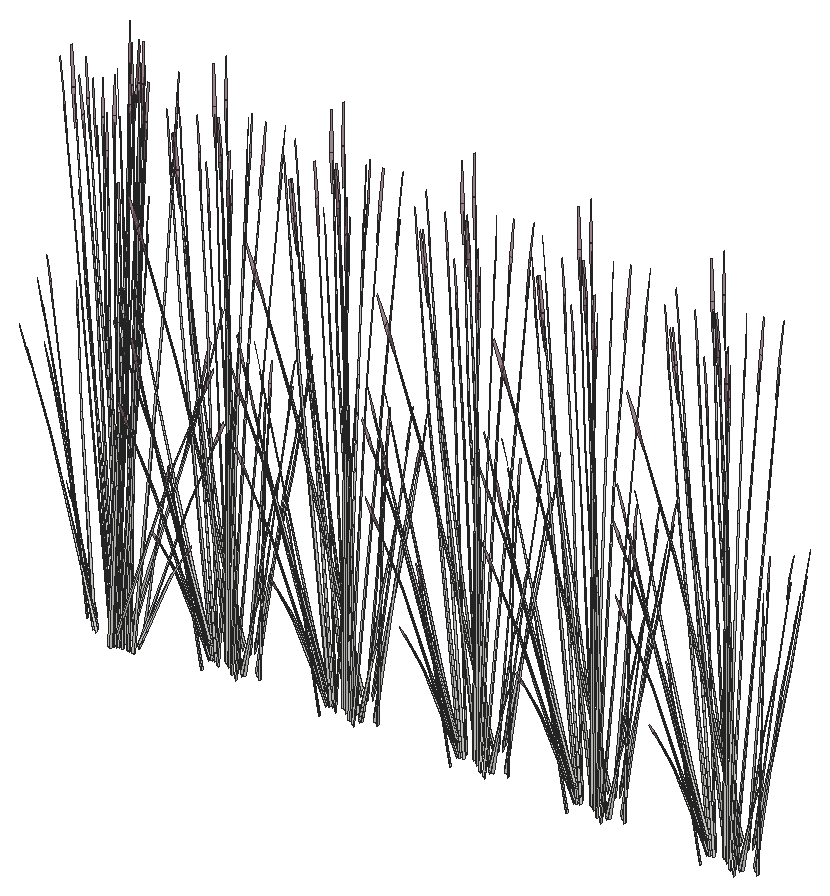
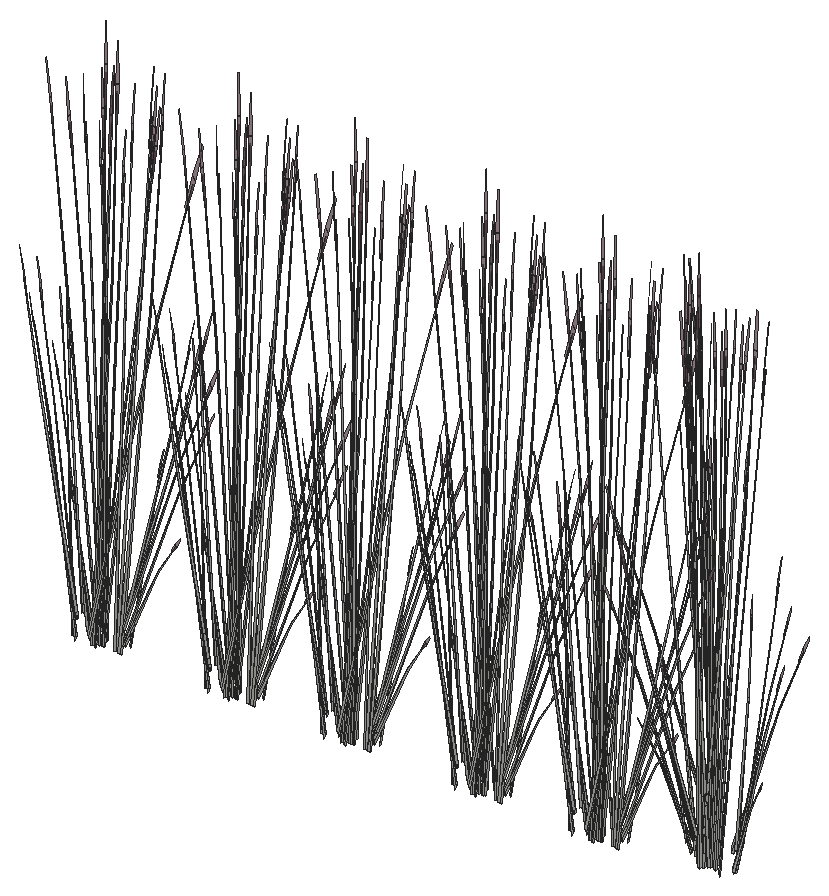
# SketchUp Ruby script. Lengths in inches.
U = 1.inch
M = Sketchup.active_model
def pt(a) = Geom::Point3d.new(a.map { |v| v * U })
def face(e, loops, mat)
  f = e.add_face(loops[0].map { |a| pt(a) })
  loops[1..].each { |l| e.add_face(l.map { |a| pt(a) }).erase! }
  f.material = f.back_material = mat if mat
  f
end
# faces: each face lists its corners as indices into pts; further lists are holes
def faces(e, pts, list, mat = nil) = list.each { |f| face(e, (f[0].is_a?(Array) ? f : [f]).map { |l| l.map { |i| pts[i] } }, mat) }
# xy, xz, yz: faces in a plane at the given z, y or x. An outline is a flat list of corners, or four numbers for a rectangle; further outlines are holes
def ring(l) = l.size == 4 ? [[l[0], l[1]], [l[2], l[1]], [l[2], l[3]], [l[0], l[3]]] : l.each_slice(2).to_a
def flat(e, list, mat, &to3) = list.each { |f| face(e, (f[0].is_a?(Array) ? f : [f]).map { |l| ring(l).map { |u, v| to3.(u, v) } }, mat) }
def xy(e, z, list, mat = nil) = flat(e, list, mat) { |x, y| [x, y, z] }
def xz(e, y, list, mat = nil) = flat(e, list, mat) { |x, z| [x, y, z] }
def yz(e, x, list, mat = nil) = flat(e, list, mat) { |y, z| [x, y, z] }
def lines(e, pts, list) = list.each { |a, b| e.add_line(pt(pts[a]), pt(pts[b])) }
# prism: a flat outline (further loops are holes) pulled along v
def prism(e, loops, v, mat = nil)
  f = face(e, loops, mat); d = Geom::Vector3d.new(v.map { |x| x * U })
  f.pushpull(f.normal.samedirection?(d) ? d.length : -d.length)
end
def box(e, o, s, mat = nil) = prism(e, [[o, [o[0] + s[0], o[1], o[2]], [o[0] + s[0], o[1] + s[1], o[2]], [o[0], o[1] + s[1], o[2]]]], [0, 0, s[2]], mat)
def at(x, y, z, deg = 0) = Geom::Transformation.translation(pt([x, y, z])) * Geom::Transformation.rotation(ORIGIN, Z_AXIS, deg.degrees)
def axes(o, x, y, z) = Geom::Transformation.new([*x, 0, *y, 0, *z, 0, *pt(o).to_a, 1])
def part(name) = M.definitions.add(name)
# library, detail: a bought-in or finely detailed component or shape, given as its bounding box
def library(name, o, s) = part(name).tap { |d| box(d.entities, o, s) }
def detail(e, o, s) = box(e.add_group.entities, o, s)
def put(e, d, t, mat = nil) = e.add_instance(d, t).tap { |i| i.material = mat if mat }
def group(e, t, mat = nil) = e.add_group.tap { |g| g.transformation = t; g.material = mat if mat }.entities
root = M.entities
M.materials.add("LightPink_Translucent").color = [144, 107, 117]
M.materials["LightPink_Translucent"].alpha = 0.75
c1 = part("blade")
p = [[2.15,0.21,22],[0,0.17,0],[0.09,0.45,0],[2.18,0.31,22],[2.29,0.31,22],[0.38,0.45,0],
  [2.48,0.24,33],[2.49,0.24,33],[2.48,0.22,33]]
faces(c1.entities,p,[[0,1,2,3],[4,5,2,3],[6,3,4,7],[8,0,3,6]])
c2 = part("seeds")
p = [[0.3,-0.1,1.38],[-0.01,-0.03,1.59],[-0.01,-0.03,0.03],[0.14,-0.07,-0.07],[0.29,-0.03,3],[0.15,0.01,3.11]]
faces(c2.entities,p,[[0,1,2,3],[1,0,4,5]],"LightPink_Translucent")
c3 = part("blade with seeds")
put(c3.entities,c1,at(0,0,0))
put(c3.entities,c2,axes([2.4,0.25,30.99],[1.5799,-0.05474,1.17369],[-0.12525,1.92788,0.29478],[-0.07173,-0.02425,1.56792]))
put(root,c3,axes([230.35,456.43,399.875],[-0.20841,0.0122,1.71376],[0.13825,-0.52864,0.13857],[0.297,0.0327,0.73262]))
put(root,c3,axes([229.68,456.33,398.38],[-0.63506,-0.11347,0.49198],[0.12924,-0.64083,0.19306],[0.09281,0.06188,1.70813]))
put(root,c3,axes([229.17,457.91,398.2],[-0.16394,-0.4643,0],[0.46814,-0.1626,0],[0,0,1.54371]))
put(root,c3,axes([228.86,457.47,398.62],[-0.09693,0.48062,0.1448],[-0.47357,-0.08343,-0.41347],[-0.08619,-0.04935,1.26744]))
put(root,c3,axes([240.53,461.875,399.33],[0.4342,0.21716,1.51261],[-0.42537,0.46784,0.59816],[-0.19053,-0.27728,1.26806]))
put(root,c3,axes([254.24,461.875,399.33],[0.4342,0.21716,1.51261],[-0.42537,0.46784,0.59816],[-0.19053,-0.27728,1.26806]))
put(root,c3,axes([269.49,461.875,399.33],[0.4342,0.21716,1.51261],[-0.42537,0.46784,0.59816],[-0.19053,-0.27728,1.26806]))
put(root,c3,axes([283.1,461.875,399.33],[0.4342,0.21716,1.51261],[-0.42537,0.46784,0.59816],[-0.19053,-0.27728,1.26806]))
put(root,c3,axes([298.63,461.875,399.33],[0.4342,0.21716,1.51261],[-0.42537,0.46784,0.59816],[-0.19053,-0.27728,1.26806]))
put(root,c3,axes([229.78,457.85,398.18],[0.5275,-0.18273,-0.19198],[0.18536,0.52636,0.00008],[0.05823,-0.0202,1.73897]))
put(root,c3,axes([229.97,458.07,398.47],[0.14515,-0.53522,0.17642],[0.53115,0.15146,0.35086],[-0.09175,0.00261,1.60407]))
put(root,c3,axes([242.61,459.71,398.59],[-0.1795,-0.01595,1.43002],[-0.18389,-0.42791,-0.30754],[0.22051,-0.12105,0.61141]))
put(root,c3,axes([256.32,459.71,398.59],[-0.1795,-0.01595,1.43002],[-0.18389,-0.42791,-0.30754],[0.22051,-0.12105,0.61141]))
put(root,c3,axes([271.57,459.71,398.59],[-0.1795,-0.01595,1.43002],[-0.18389,-0.42791,-0.30754],[0.22051,-0.12105,0.61141]))
put(root,c3,axes([285.18,459.71,398.59],[-0.1795,-0.01595,1.43002],[-0.18389,-0.42791,-0.30754],[0.22051,-0.12105,0.61141]))
put(root,c3,axes([300.71,459.71,398.59],[-0.1795,-0.01595,1.43002],[-0.18389,-0.42791,-0.30754],[0.22051,-0.12105,0.61141]))
put(root,c3,axes([229.84,456.85,398.21],[0.35073,0.34786,0],[-0.35073,0.34786,0],[0,0,1.69266]))
put(root,c3,axes([227.85,456.2,399.34],[0.14282,-0.0779,1.77064],[0.04925,0.54394,0.13857],[-0.30935,0.07218,0.63284]))
put(root,c3,axes([230.79,456.7,398.47],[-0.39477,-0.39228,0.17642],[0.39783,-0.38049,0.35086],[-0.0436,0.08011,1.60407]))
put(root,c3,axes([232.375,457.06,398.77],[-0.31044,0.08891,1.1486],[0.14613,-0.36744,0.84392],[0.16469,0.02514,0.25299]))
put(root,c3,axes([242.82,458.92,398.77],[-0.16736,0.27414,1.1486],[-0.14385,-0.36832,0.84392],[0.13822,-0.09229,0.25299]))
put(root,c3,axes([256.53,458.92,398.77],[-0.16736,0.27414,1.1486],[-0.14385,-0.36832,0.84392],[0.13822,-0.09229,0.25299]))
put(root,c3,axes([271.77,458.92,398.77],[-0.16736,0.27414,1.1486],[-0.14385,-0.36832,0.84392],[0.13822,-0.09229,0.25299]))
put(root,c3,axes([285.39,458.92,398.77],[-0.16736,0.27414,1.1486],[-0.14385,-0.36832,0.84392],[0.13822,-0.09229,0.25299]))
put(root,c3,axes([300.92,458.92,398.77],[-0.16736,0.27414,1.1486],[-0.14385,-0.36832,0.84392],[0.13822,-0.09229,0.25299]))
put(root,c3,axes([229.05,458.12,398.2],[-0.50654,-0.24178,0],[0.24378,-0.50239,0],[0,0,1.62707]))
put(root,c3,axes([229.47,457.48,398.46],[-0.49063,-0.43346,-0.25192],[0.41285,-0.48673,0.5513],[-0.13212,0.05071,1.68216]))
put(root,c3,axes([228.18,458.31,398.48],[0.47024,0.26927,0.49651],[-0.28107,0.48284,0],[-0.1071,-0.06133,1.57504]))
put(root,c3,axes([242.58,459.95,400.53],[0.43736,-0.07697,-0.35414],[0.11549,0.43998,0.4572],[0.12533,-0.11818,0.87481]))
put(root,c3,axes([256.29,459.95,400.53],[0.43736,-0.07697,-0.35414],[0.11549,0.43998,0.4572],[0.12533,-0.11818,0.87481]))
put(root,c3,axes([271.54,459.95,400.53],[0.43736,-0.07697,-0.35414],[0.11549,0.43998,0.4572],[0.12533,-0.11818,0.87481]))
put(root,c3,axes([285.15,459.95,400.53],[0.43736,-0.07697,-0.35414],[0.11549,0.43998,0.4572],[0.12533,-0.11818,0.87481]))
put(root,c3,axes([300.68,459.95,400.53],[0.43736,-0.07697,-0.35414],[0.11549,0.43998,0.4572],[0.12533,-0.11818,0.87481]))
put(root,c3,axes([229.84,456.45,398.72],[0.24378,-0.48527,0.44739],[0.50654,0.23354,-0.21531],[0,0.11186,1.43643]))
put(root,c3,axes([238.33,459.35,400.53],[-0.28589,-0.33718,-0.35414],[0.32644,-0.31919,0.4572],[-0.16586,-0.04856,0.87481]))
put(root,c3,axes([252.04,459.35,400.53],[-0.28589,-0.33718,-0.35414],[0.32644,-0.31919,0.4572],[-0.16586,-0.04856,0.87481]))
put(root,c3,axes([267.28,459.35,400.53],[-0.28589,-0.33718,-0.35414],[0.32644,-0.31919,0.4572],[-0.16586,-0.04856,0.87481]))
put(root,c3,axes([280.9,459.35,400.53],[-0.28589,-0.33718,-0.35414],[0.32644,-0.31919,0.4572],[-0.16586,-0.04856,0.87481]))
put(root,c3,axes([296.43,459.35,400.53],[-0.28589,-0.33718,-0.35414],[0.32644,-0.31919,0.4572],[-0.16586,-0.04856,0.87481]))
put(root,c3,axes([229.75,456.72,398.29],[0,0.62282,-0.05637],[-0.62828,0,0],[0,0.01957,1.79368]))
put(root,c3,axes([240.01,460.35,398.67],[-0.05855,-0.61451,-0.29095],[0.60981,-0.03716,-0.50002],[0.10738,-0.08185,1.59708]))
put(root,c3,axes([253.72,460.35,398.67],[-0.05855,-0.61451,-0.29095],[0.60981,-0.03716,-0.50002],[0.10738,-0.08185,1.59708]))
put(root,c3,axes([268.97,460.35,398.67],[-0.05855,-0.61451,-0.29095],[0.60981,-0.03716,-0.50002],[0.10738,-0.08185,1.59708]))
put(root,c3,axes([282.58,460.35,398.67],[-0.05855,-0.61451,-0.29095],[0.60981,-0.03716,-0.50002],[0.10738,-0.08185,1.59708]))
put(root,c3,axes([298.11,460.35,398.67],[-0.05855,-0.61451,-0.29095],[0.60981,-0.03716,-0.50002],[0.10738,-0.08185,1.59708]))
put(root,c3,axes([226.87,456.5,400.68],[-0.13612,0.48987,-0.51099],[-0.46669,-0.16791,-0.3958],[-0.1879,0.04492,0.97773]))
put(root,c3,axes([231.83,458.19,399.93],[-0.09617,-0.45271,-0.03492],[0.45453,-0.10408,-0.15832],[0.09492,0.0287,0.52218]))
put(root,c3,axes([227.91,458.59,398.375],[-0.31414,0.53965,0],[-0.52557,-0.30095,-0.51607],[-0.1197,-0.06854,1.63711]))
put(root,c3,axes([238.36,458.77,398.13],[-0.14494,0.43975,-0.03893],[-0.4461,-0.13527,-0.17649],[-0.06773,-0.07192,0.58215]))
put(root,c3,axes([252.07,458.77,398.13],[-0.14494,0.43975,-0.03893],[-0.4461,-0.13527,-0.17649],[-0.06773,-0.07192,0.58215]))
put(root,c3,axes([267.3125,458.77,398.13],[-0.14494,0.43975,-0.03893],[-0.4461,-0.13527,-0.17649],[-0.06773,-0.07192,0.58215]))
put(root,c3,axes([280.93,458.77,398.13],[-0.14494,0.43975,-0.03893],[-0.4461,-0.13527,-0.17649],[-0.06773,-0.07192,0.58215]))
put(root,c3,axes([296.46,458.77,398.13],[-0.14494,0.43975,-0.03893],[-0.4461,-0.13527,-0.17649],[-0.06773,-0.07192,0.58215]))
put(root,c3,axes([239.73,461,398.67],[-0.56585,-0.25696,-0.29095],[0.27246,-0.54236,-0.50002],[-0.01778,-0.13316,1.59708]))
put(root,c3,axes([253.4375,461,398.67],[-0.56585,-0.25696,-0.29095],[0.27246,-0.54236,-0.50002],[-0.01778,-0.13316,1.59708]))
put(root,c3,axes([268.68,461,398.67],[-0.56585,-0.25696,-0.29095],[0.27246,-0.54236,-0.50002],[-0.01778,-0.13316,1.59708]))
put(root,c3,axes([282.3,461,398.67],[-0.56585,-0.25696,-0.29095],[0.27246,-0.54236,-0.50002],[-0.01778,-0.13316,1.59708]))
put(root,c3,axes([297.83,461,398.67],[-0.56585,-0.25696,-0.29095],[0.27246,-0.54236,-0.50002],[-0.01778,-0.13316,1.59708]))
put(root,c3,axes([231.12,456.72,398.48],[0,-0.53854,0.49651],[0.56215,0,0],[0,0.12266,1.57504]))
put(root,c3,axes([238.12,460.78,398.375],[-0.62828,0,0],[0,-0.6019,-0.51607],[0,-0.13709,1.63711]))
put(root,c3,axes([251.83,460.78,398.375],[-0.62828,0,0],[0,-0.6019,-0.51607],[0,-0.13709,1.63711]))
put(root,c3,axes([267.07,460.78,398.375],[-0.62828,0,0],[0,-0.6019,-0.51607],[0,-0.13709,1.63711]))
put(root,c3,axes([280.6875,460.78,398.375],[-0.62828,0,0],[0,-0.6019,-0.51607],[0,-0.13709,1.63711]))
put(root,c3,axes([296.22,460.78,398.375],[-0.62828,0,0],[0,-0.6019,-0.51607],[0,-0.13709,1.63711]))
put(root,c3,axes([229.71,457.12,398.72],[0.54562,-0.03324,0.44739],[0.04934,0.55185,-0.21531],[-0.09768,0.05593,1.43643]))
put(root,c3,axes([230.05,456.56,398.62],[0.46814,-0.15705,0.1448],[0.16394,0.44848,-0.41347],[0,0.0987,1.26744]))
put(root,c3,axes([238.23,459.71,398.59],[0.0981,0.14994,1.43002],[-0.22605,0.40756,-0.30754],[-0.23211,-0.09741,0.61141]))
put(root,c3,axes([251.93,459.71,398.59],[0.0981,0.14994,1.43002],[-0.22605,0.40756,-0.30754],[-0.23211,-0.09741,0.61141]))
put(root,c3,axes([267.18,459.71,398.59],[0.0981,0.14994,1.43002],[-0.22605,0.40756,-0.30754],[-0.23211,-0.09741,0.61141]))
put(root,c3,axes([280.79,459.71,398.59],[0.0981,0.14994,1.43002],[-0.22605,0.40756,-0.30754],[-0.23211,-0.09741,0.61141]))
put(root,c3,axes([296.33,459.71,398.59],[0.0981,0.14994,1.43002],[-0.22605,0.40756,-0.30754],[-0.23211,-0.09741,0.61141]))
put(root,c3,axes([238.63,459.57,400.98],[-0.50227,-0.01297,-0.71045],[0.03373,-0.54602,0.08574],[-0.21278,-0.05762,1.00501]))
put(root,c3,axes([252.34,459.57,400.98],[-0.50227,-0.01297,-0.71045],[0.03373,-0.54602,0.08574],[-0.21278,-0.05762,1.00501]))
put(root,c3,axes([267.59,459.57,400.98],[-0.50227,-0.01297,-0.71045],[0.03373,-0.54602,0.08574],[-0.21278,-0.05762,1.00501]))
put(root,c3,axes([281.2,459.57,400.98],[-0.50227,-0.01297,-0.71045],[0.03373,-0.54602,0.08574],[-0.21278,-0.05762,1.00501]))
put(root,c3,axes([296.73,459.57,400.98],[-0.50227,-0.01297,-0.71045],[0.03373,-0.54602,0.08574],[-0.21278,-0.05762,1.00501]))
put(root,c3,axes([231.79,457.65,398.59],[-0.12101,-0.13245,1.43002],[0.15744,-0.43816,-0.30754],[0.24483,0.05936,0.61141]))
put(root,c3,axes([229.63,458.13,398.2],[0.50654,0.24178,0],[-0.24378,0.50239,0],[0,0,1.74954]))
put(root,c3,axes([229.83,458.67,398.19],[-0.31023,-0.54153,-0.05142],[0.52557,-0.30095,0.51607],[-0.12951,0.05156,1.6363]))
put(root,c3,axes([229.72,457.36,398.62],[0.37121,0.32357,0.1448],[-0.30963,0.36505,-0.41347],[-0.08619,0.04935,1.26744]))
put(root,c3,axes([226.85,456.75,399.875],[0.17434,-0.11391,1.71376],[0.14677,0.52637,0.13857],[-0.27369,0.11897,0.73262]))
put(root,c3,axes([238.61,460.625,398.33],[-0.46736,0.45277,0.30756],[-0.46764,-0.44801,-0.36492],[-0.01632,-0.12858,1.64885]))
put(root,c3,axes([252.3125,460.625,398.33],[-0.46736,0.45277,0.30756],[-0.46764,-0.44801,-0.36492],[-0.01632,-0.12858,1.64885]))
put(root,c3,axes([267.5625,460.625,398.33],[-0.46736,0.45277,0.30756],[-0.46764,-0.44801,-0.36492],[-0.01632,-0.12858,1.64885]))
put(root,c3,axes([281.17,460.625,398.33],[-0.46736,0.45277,0.30756],[-0.46764,-0.44801,-0.36492],[-0.01632,-0.12858,1.64885]))
put(root,c3,axes([296.71,460.625,398.33],[-0.46736,0.45277,0.30756],[-0.46764,-0.44801,-0.36492],[-0.01632,-0.12858,1.64885]))
put(root,c3,axes([240.09,460.83,398.43],[0.56613,0.26102,0.24065],[-0.27246,0.54236,0.50002],[0,-0.12502,1.60543]))
put(root,c3,axes([253.8,460.83,398.43],[0.56613,0.26102,0.24065],[-0.27246,0.54236,0.50002],[0,-0.12502,1.60543]))
put(root,c3,axes([269.05,460.83,398.43],[0.56613,0.26102,0.24065],[-0.27246,0.54236,0.50002],[0,-0.12502,1.60543]))
put(root,c3,axes([282.66,460.83,398.43],[0.56613,0.26102,0.24065],[-0.27246,0.54236,0.50002],[0,-0.12502,1.60543]))
put(root,c3,axes([298.19,460.83,398.43],[0.56613,0.26102,0.24065],[-0.27246,0.54236,0.50002],[0,-0.12502,1.60543]))
put(root,c3,axes([239.87,461.57,398.4375],[0.13317,-0.63814,-0.23429],[0.63143,0.11124,0.51271],[-0.11033,-0.08813,1.5644]))
put(root,c3,axes([253.58,461.57,398.4375],[0.13317,-0.63814,-0.23429],[0.63143,0.11124,0.51271],[-0.11033,-0.08813,1.5644]))
put(root,c3,axes([268.83,461.57,398.4375],[0.13317,-0.63814,-0.23429],[0.63143,0.11124,0.51271],[-0.11033,-0.08813,1.5644]))
put(root,c3,axes([282.44,461.57,398.4375],[0.13317,-0.63814,-0.23429],[0.63143,0.11124,0.51271],[-0.11033,-0.08813,1.5644]))
put(root,c3,axes([297.97,461.57,398.4375],[0.13317,-0.63814,-0.23429],[0.63143,0.11124,0.51271],[-0.11033,-0.08813,1.5644]))
put(root,c3,axes([230.68,457.92,400.98],[0.50227,0.01297,-0.71045],[-0.03373,0.54602,0.08574],[0.21278,0.05762,1.00501]))
put(root,c3,axes([238.46,459.68,400.68],[-0.36484,0.35674,-0.51099],[-0.31952,-0.37685,-0.3958],[-0.18537,-0.05428,0.97773]))
put(root,c3,axes([252.17,459.68,400.68],[-0.36484,0.35674,-0.51099],[-0.31952,-0.37685,-0.3958],[-0.18537,-0.05428,0.97773]))
put(root,c3,axes([267.42,459.68,400.68],[-0.36484,0.35674,-0.51099],[-0.31952,-0.37685,-0.3958],[-0.18537,-0.05428,0.97773]))
put(root,c3,axes([281.03,459.68,400.68],[-0.36484,0.35674,-0.51099],[-0.31952,-0.37685,-0.3958],[-0.18537,-0.05428,0.97773]))
put(root,c3,axes([296.5625,459.68,400.68],[-0.36484,0.35674,-0.51099],[-0.31952,-0.37685,-0.3958],[-0.18537,-0.05428,0.97773]))
put(root,c3,axes([230.12,458.35,398.48],[0.47024,-0.26927,0.49651],[0.28107,0.48284,0],[-0.1071,0.06133,1.57504]))
put(root,c3,axes([237.64,460.16,398.77],[0.32078,-0.03854,1.1486],[-0.20348,0.33954,0.84392],[-0.15852,-0.05093,0.25299]))
put(root,c3,axes([251.35,460.16,398.77],[0.32078,-0.03854,1.1486],[-0.20348,0.33954,0.84392],[-0.15852,-0.05093,0.25299]))
put(root,c3,axes([266.6,460.16,398.77],[0.32078,-0.03854,1.1486],[-0.20348,0.33954,0.84392],[-0.15852,-0.05093,0.25299]))
put(root,c3,axes([280.21,460.16,398.77],[0.32078,-0.03854,1.1486],[-0.20348,0.33954,0.84392],[-0.15852,-0.05093,0.25299]))
put(root,c3,axes([295.74,460.16,398.77],[0.32078,-0.03854,1.1486],[-0.20348,0.33954,0.84392],[-0.15852,-0.05093,0.25299]))
put(root,c3,axes([229.45,457.93,398.29],[0.21845,0.61869,-0.06012],[-0.62418,0.21679,0],[0.00763,0.02161,1.72173]))
put(root,c3,axes([226.31,457.65,398.59],[0.17462,0.04421,1.43002],[0.11254,0.45156,-0.30754],[-0.23719,0.08453,0.61141]))
put(root,c3,axes([239.91,460.47,398.72],[-0.54562,0.03324,0.44739],[-0.04934,-0.55185,-0.21531],[0.09768,-0.05593,1.43643]))
put(root,c3,axes([253.62,460.47,398.72],[-0.54562,0.03324,0.44739],[-0.04934,-0.55185,-0.21531],[0.09768,-0.05593,1.43643]))
put(root,c3,axes([268.86,460.47,398.72],[-0.54562,0.03324,0.44739],[-0.04934,-0.55185,-0.21531],[0.09768,-0.05593,1.43643]))
put(root,c3,axes([282.48,460.47,398.72],[-0.54562,0.03324,0.44739],[-0.04934,-0.55185,-0.21531],[0.09768,-0.05593,1.43643]))
put(root,c3,axes([298.01,460.47,398.72],[-0.54562,0.03324,0.44739],[-0.04934,-0.55185,-0.21531],[0.09768,-0.05593,1.43643]))
put(root,c3,axes([231.5,456.81,398.375],[0.62828,0,0],[0,0.6019,-0.51607],[0,0.13709,1.63711]))
put(root,c3,axes([238.5,460.875,398.48],[0,0.53854,0.49651],[-0.56215,0,0],[0,-0.12266,1.57504]))
put(root,c3,axes([252.21,460.875,398.48],[0,0.53854,0.49651],[-0.56215,0,0],[0,-0.12266,1.57504]))
put(root,c3,axes([267.46,460.875,398.48],[0,0.53854,0.49651],[-0.56215,0,0],[0,-0.12266,1.57504]))
put(root,c3,axes([281.07,460.875,398.48],[0,0.53854,0.49651],[-0.56215,0,0],[0,-0.12266,1.57504]))
put(root,c3,axes([296.6,460.875,398.48],[0,0.53854,0.49651],[-0.56215,0,0],[0,-0.12266,1.57504]))
put(root,c3,axes([231.25,457.12,398.2],[-0.62797,-0.00431,-0.04976],[0,-0.6019,0.49943],[-0.01973,0.13702,1.58352]))
put(root,c3,axes([242.45,460.99,400.68],[0.13612,-0.48987,-0.51099],[0.46669,0.16791,-0.3958],[0.1879,-0.04492,0.97773]))
put(root,c3,axes([256.15,460.99,400.68],[0.13612,-0.48987,-0.51099],[0.46669,0.16791,-0.3958],[0.1879,-0.04492,0.97773]))
put(root,c3,axes([271.4,460.99,400.68],[0.13612,-0.48987,-0.51099],[0.46669,0.16791,-0.3958],[0.1879,-0.04492,0.97773]))
put(root,c3,axes([285.02,460.99,400.68],[0.13612,-0.48987,-0.51099],[0.46669,0.16791,-0.3958],[0.1879,-0.04492,0.97773]))
put(root,c3,axes([300.55,460.99,400.68],[0.13612,-0.48987,-0.51099],[0.46669,0.16791,-0.3958],[0.1879,-0.04492,0.97773]))
put(root,c3,axes([241.71,459,398.375],[0.31414,-0.53965,0],[0.52557,0.30095,-0.51607],[0.1197,0.06854,1.63711]))
put(root,c3,axes([255.42,459,398.375],[0.31414,-0.53965,0],[0.52557,0.30095,-0.51607],[0.1197,0.06854,1.63711]))
put(root,c3,axes([270.66,459,398.375],[0.31414,-0.53965,0],[0.52557,0.30095,-0.51607],[0.1197,0.06854,1.63711]))
put(root,c3,axes([284.28,459,398.375],[0.31414,-0.53965,0],[0.52557,0.30095,-0.51607],[0.1197,0.06854,1.63711]))
put(root,c3,axes([299.81,459,398.375],[0.31414,-0.53965,0],[0.52557,0.30095,-0.51607],[0.1197,0.06854,1.63711]))
put(root,c3,axes([238.01,460.07,399.875],[0.20841,-0.0122,1.71376],[-0.13825,0.52864,0.13857],[-0.297,-0.0327,0.73262]))
put(root,c3,axes([251.72,460.07,399.875],[0.20841,-0.0122,1.71376],[-0.13825,0.52864,0.13857],[-0.297,-0.0327,0.73262]))
put(root,c3,axes([266.96,460.07,399.875],[0.20841,-0.0122,1.71376],[-0.13825,0.52864,0.13857],[-0.297,-0.0327,0.73262]))
put(root,c3,axes([280.58,460.07,399.875],[0.20841,-0.0122,1.71376],[-0.13825,0.52864,0.13857],[-0.297,-0.0327,0.73262]))
put(root,c3,axes([296.11,460.07,399.875],[0.20841,-0.0122,1.71376],[-0.13825,0.52864,0.13857],[-0.297,-0.0327,0.73262]))
put(root,c3,axes([225.94,458.59,398.77],[0.2094,-0.24408,1.1486],[0.08263,0.38639,0.84392],[-0.15132,0.06919,0.25299]))
put(root,c3,axes([230.98,458.14,400.53],[0.28589,0.33718,-0.35414],[-0.32644,0.31919,0.4572],[0.16586,0.04856,0.87481]))
put(root,c3,axes([239.89,460.67,398.36],[0.21845,0.6022,0.45755],[-0.62418,0.20941,0.17955],[0.00763,-0.11065,1.58856]))
put(root,c3,axes([253.6,460.67,398.36],[0.21845,0.6022,0.45755],[-0.62418,0.20941,0.17955],[0.00763,-0.11065,1.58856]))
put(root,c3,axes([268.85,460.67,398.36],[0.21845,0.6022,0.45755],[-0.62418,0.20941,0.17955],[0.00763,-0.11065,1.58856]))
put(root,c3,axes([282.46,460.67,398.36],[0.21845,0.6022,0.45755],[-0.62418,0.20941,0.17955],[0.00763,-0.11065,1.58856]))
put(root,c3,axes([297.99,460.67,398.36],[0.21845,0.6022,0.45755],[-0.62418,0.20941,0.17955],[0.00763,-0.11065,1.58856]))
put(root,c3,axes([226.73,457.54,400.53],[-0.43736,0.07697,-0.35414],[-0.11549,-0.43998,0.4572],[-0.12533,0.11818,0.87481]))
put(root,c3,axes([242.94,461.13,397.98],[-0.32361,0.06463,1.41583],[-0.05151,-0.51444,0.08104],[0.22666,-0.07786,0.80566]))
put(root,c3,axes([256.65,461.13,397.98],[-0.32361,0.06463,1.41583],[-0.05151,-0.51444,0.08104],[0.22666,-0.07786,0.80566]))
put(root,c3,axes([271.9,461.13,397.98],[-0.32361,0.06463,1.41583],[-0.05151,-0.51444,0.08104],[0.22666,-0.07786,0.80566]))
put(root,c3,axes([285.51,461.13,397.98],[-0.32361,0.06463,1.41583],[-0.05151,-0.51444,0.08104],[0.22666,-0.07786,0.80566]))
put(root,c3,axes([301.04,461.13,397.98],[-0.32361,0.06463,1.41583],[-0.05151,-0.51444,0.08104],[0.22666,-0.07786,0.80566]))
put(root,c3,axes([243.53,460.68,398.26],[-0.31151,-0.34437,-0.06488],[0.34117,-0.31553,-0.29416],[0.09667,-0.02221,0.97024]))
put(root,c3,axes([257.24,460.68,398.26],[-0.31151,-0.34437,-0.06488],[0.34117,-0.31553,-0.29416],[0.09667,-0.02221,0.97024]))
put(root,c3,axes([272.49,460.68,398.26],[-0.31151,-0.34437,-0.06488],[0.34117,-0.31553,-0.29416],[0.09667,-0.02221,0.97024]))
put(root,c3,axes([286.1,460.68,398.26],[-0.31151,-0.34437,-0.06488],[0.34117,-0.31553,-0.29416],[0.09667,-0.02221,0.97024]))
put(root,c3,axes([301.63,460.68,398.26],[-0.31151,-0.34437,-0.06488],[0.34117,-0.31553,-0.29416],[0.09667,-0.02221,0.97024]))
put(root,c3,axes([239.78,461.14,398.72],[-0.24378,0.48527,0.44739],[-0.50654,-0.23354,-0.21531],[0,-0.11186,1.43643]))
put(root,c3,axes([253.49,461.14,398.72],[-0.24378,0.48527,0.44739],[-0.50654,-0.23354,-0.21531],[0,-0.11186,1.43643]))
put(root,c3,axes([268.74,461.14,398.72],[-0.24378,0.48527,0.44739],[-0.50654,-0.23354,-0.21531],[0,-0.11186,1.43643]))
put(root,c3,axes([282.35,461.14,398.72],[-0.24378,0.48527,0.44739],[-0.50654,-0.23354,-0.21531],[0,-0.11186,1.43643]))
put(root,c3,axes([297.88,461.14,398.72],[-0.24378,0.48527,0.44739],[-0.50654,-0.23354,-0.21531],[0,-0.11186,1.43643]))
put(root,c3,axes([240.68,460.72,398.21],[0,-0.62313,0],[0.62828,0,0],[0,0,1.79456]))
put(root,c3,axes([254.38,460.72,398.21],[0,-0.62313,0],[0.62828,0,0],[0,0,1.79456]))
put(root,c3,axes([269.63,460.72,398.21],[0,-0.62313,0],[0.62828,0,0],[0,0,1.79456]))
put(root,c3,axes([283.24,460.72,398.21],[0,-0.62313,0],[0.62828,0,0],[0,0,1.79456]))
put(root,c3,axes([298.77,460.72,398.21],[0,-0.62313,0],[0.62828,0,0],[0,0,1.79456]))
put(root,c3,axes([241.4375,459.28,398.48],[-0.47024,-0.26927,0.49651],[0.28107,-0.48284,0],[0.1071,0.06133,1.57504]))
put(root,c3,axes([255.14,459.28,398.48],[-0.47024,-0.26927,0.49651],[0.28107,-0.48284,0],[0.1071,0.06133,1.57504]))
put(root,c3,axes([270.39,459.28,398.48],[-0.47024,-0.26927,0.49651],[0.28107,-0.48284,0],[0.1071,0.06133,1.57504]))
put(root,c3,axes([284.01,459.28,398.48],[-0.47024,-0.26927,0.49651],[0.28107,-0.48284,0],[0.1071,0.06133,1.57504]))
put(root,c3,axes([299.54,459.28,398.48],[-0.47024,-0.26927,0.49651],[0.28107,-0.48284,0],[0.1071,0.06133,1.57504]))
put(root,c3,axes([242.36,461.17,400.98],[0.44151,-0.23785,-0.71045],[0.24605,0.4896,0.08574],[0.21333,-0.05562,1.00501]))
put(root,c3,axes([256.06,461.17,400.98],[0.44151,-0.23785,-0.71045],[0.24605,0.4896,0.08574],[0.21333,-0.05562,1.00501]))
put(root,c3,axes([271.3125,461.17,400.98],[0.44151,-0.23785,-0.71045],[0.24605,0.4896,0.08574],[0.21333,-0.05562,1.00501]))
put(root,c3,axes([284.93,461.17,400.98],[0.44151,-0.23785,-0.71045],[0.24605,0.4896,0.08574],[0.21333,-0.05562,1.00501]))
put(root,c3,axes([300.46,461.17,400.98],[0.44151,-0.23785,-0.71045],[0.24605,0.4896,0.08574],[0.21333,-0.05562,1.00501]))
put(root,c3,axes([240.38,460.33,398.36],[-0.4166,0.48873,0.45755],[-0.49494,-0.43142,0.17955],[0.10044,-0.04877,1.58856]))
put(root,c3,axes([254.09,460.33,398.36],[-0.4166,0.48873,0.45755],[-0.49494,-0.43142,0.17955],[0.10044,-0.04877,1.58856]))
put(root,c3,axes([269.33,460.33,398.36],[-0.4166,0.48873,0.45755],[-0.49494,-0.43142,0.17955],[0.10044,-0.04877,1.58856]))
put(root,c3,axes([282.95,460.33,398.36],[-0.4166,0.48873,0.45755],[-0.49494,-0.43142,0.17955],[0.10044,-0.04877,1.58856]))
put(root,c3,axes([298.48,460.33,398.36],[-0.4166,0.48873,0.45755],[-0.49494,-0.43142,0.17955],[0.10044,-0.04877,1.58856]))
put(root,c3,axes([240.83,461.2,398.3],[-0.46736,-0.46353,-0.06131],[0.46764,-0.46381,0],[-0.01632,-0.01619,1.75571]))
put(root,c3,axes([254.54,461.2,398.3],[-0.46736,-0.46353,-0.06131],[0.46764,-0.46381,0],[-0.01632,-0.01619,1.75571]))
put(root,c3,axes([269.79,461.2,398.3],[-0.46736,-0.46353,-0.06131],[0.46764,-0.46381,0],[-0.01632,-0.01619,1.75571]))
put(root,c3,axes([283.4,461.2,398.3],[-0.46736,-0.46353,-0.06131],[0.46764,-0.46381,0],[-0.01632,-0.01619,1.75571]))
put(root,c3,axes([298.93,461.2,398.3],[-0.46736,-0.46353,-0.06131],[0.46764,-0.46381,0],[-0.01632,-0.01619,1.75571]))
put(root,c3,axes([229.84,458.39,398.33],[0.62903,0.17504,0.30756],[-0.15737,0.62568,-0.36492],[-0.10411,0.07831,1.64885]))
put(root,c3,axes([239.65,459.52,398.47],[-0.14515,0.53522,0.17642],[-0.53115,-0.15146,0.35086],[0.09175,-0.00261,1.60407]))
put(root,c3,axes([253.36,459.52,398.47],[-0.14515,0.53522,0.17642],[-0.53115,-0.15146,0.35086],[0.09175,-0.00261,1.60407]))
